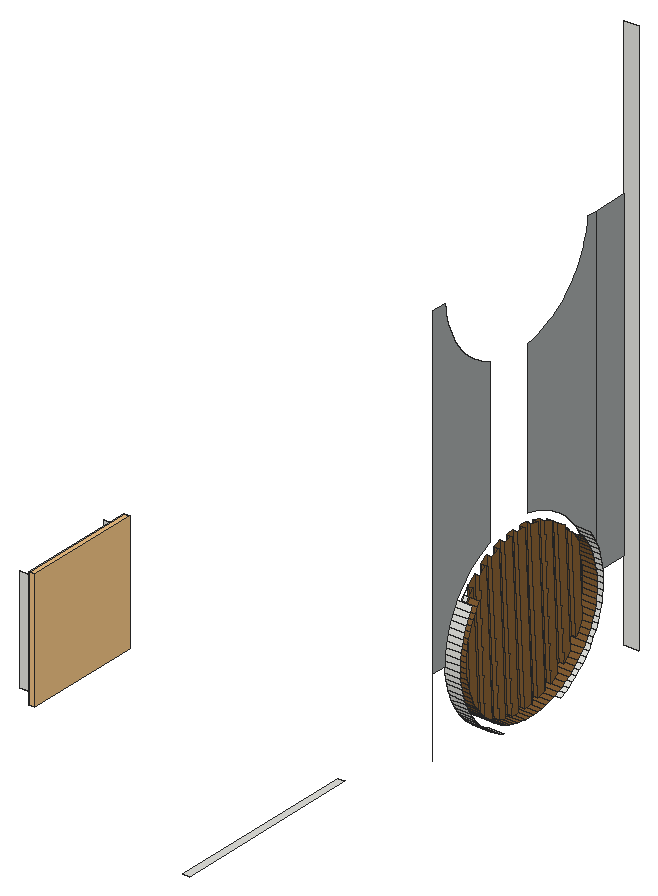
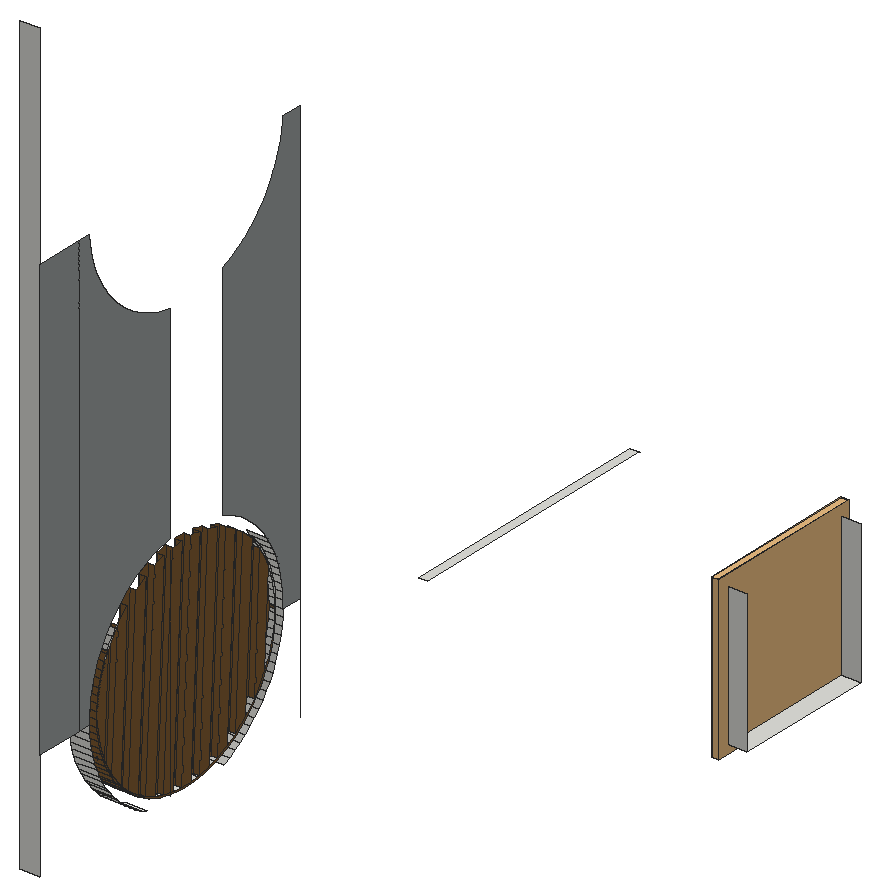
# SketchUp Ruby script. Lengths in inches.
U = 1.inch
M = Sketchup.active_model
def pt(a) = Geom::Point3d.new(a.map { |v| v * U })
def face(e, loops, mat)
  f = e.add_face(loops[0].map { |a| pt(a) })
  loops[1..].each { |l| e.add_face(l.map { |a| pt(a) }).erase! }
  f.material = f.back_material = mat if mat
  f
end
# faces: each face lists its corners as indices into pts; further lists are holes
def faces(e, pts, list, mat = nil) = list.each { |f| face(e, (f[0].is_a?(Array) ? f : [f]).map { |l| l.map { |i| pts[i] } }, mat) }
# xy, xz, yz: faces in a plane at the given z, y or x. An outline is a flat list of corners, or four numbers for a rectangle; further outlines are holes
def ring(l) = l.size == 4 ? [[l[0], l[1]], [l[2], l[1]], [l[2], l[3]], [l[0], l[3]]] : l.each_slice(2).to_a
def flat(e, list, mat, &to3) = list.each { |f| face(e, (f[0].is_a?(Array) ? f : [f]).map { |l| ring(l).map { |u, v| to3.(u, v) } }, mat) }
def xy(e, z, list, mat = nil) = flat(e, list, mat) { |x, y| [x, y, z] }
def xz(e, y, list, mat = nil) = flat(e, list, mat) { |x, z| [x, y, z] }
def yz(e, x, list, mat = nil) = flat(e, list, mat) { |y, z| [x, y, z] }
def lines(e, pts, list) = list.each { |a, b| e.add_line(pt(pts[a]), pt(pts[b])) }
# prism: a flat outline (further loops are holes) pulled along v
def prism(e, loops, v, mat = nil)
  f = face(e, loops, mat); d = Geom::Vector3d.new(v.map { |x| x * U })
  f.pushpull(f.normal.samedirection?(d) ? d.length : -d.length)
end
def box(e, o, s, mat = nil) = prism(e, [[o, [o[0] + s[0], o[1], o[2]], [o[0] + s[0], o[1] + s[1], o[2]], [o[0], o[1] + s[1], o[2]]]], [0, 0, s[2]], mat)
def at(x, y, z, deg = 0) = Geom::Transformation.translation(pt([x, y, z])) * Geom::Transformation.rotation(ORIGIN, Z_AXIS, deg.degrees)
def axes(o, x, y, z) = Geom::Transformation.new([*x, 0, *y, 0, *z, 0, *pt(o).to_a, 1])
def part(name) = M.definitions.add(name)
# library, detail: a bought-in or finely detailed component or shape, given as its bounding box
def library(name, o, s) = part(name).tap { |d| box(d.entities, o, s) }
def detail(e, o, s) = box(e.add_group.entities, o, s)
def put(e, d, t, mat = nil) = e.add_instance(d, t).tap { |i| i.material = mat if mat }
def group(e, t, mat = nil) = e.add_group.tap { |g| g.transformation = t; g.material = mat if mat }.entities
root = M.entities
M.materials.add("C08_Toffee_Ember").color = [130, 92, 50]
M.materials.add("Denim_03_1K").color = [156, 160, 160]
c1 = library("mesh-165",[-1596.32,-2661.67,-39.91],[1702.88,1739.15,82.5])
c2 = part("Group15")
put(c2.entities,c1,at(294.66,859.51,3.5))
xy(root,168,[[317.82,21,320.5,99]])
xy(root,171,[[206.5,78,212.5,120]])
xz(root,78,[[206.5,171,212.5,213]])
xz(root,120,[[206.5,171,212.5,213]])
xz(root,156.01,[[317.5,186.29,319.5,186.76]])
xz(root,243,[[317.5,153,323.5,378]])
yz(root,212.5,[[[75,168,123,216],[78,171,120,213]]])
yz(root,317.5,[[221.99,185.81,222,186.07,221.97,187.24],[156.01,186.29,156.01,186.76,156.12,188.83,156.36,190.89,156.74,192.93,157.23,194.9375,157.86,196.92,158.6,198.85,158.62,198.88,158.6,199.26,158.46,198.9375,157.73,197,157.13,195.01,156.66,192.99,156.31,190.95,156.09,188.89,156,186.82],[221.97,187.33,221.96,188.14,221.78,190.21,221.48,192.26,221.05,194.29,220.5,196.29,219.82,198.25,219.02,200.16,218.1,202.01,217.92,202.32,217.95,201.82,218.28,201.23,219.17,199.36,219.95,197.44,220.61,195.47,221.14,193.47,221.55,191.4375,221.83,189.38],[158.62,198.88,159.47,200.73,160.45,202.56,161.55,204.32,161.64,204.4375,161.62,204.84,161.34,204.44,160.26,202.67,159.3,200.83,158.6,199.26],[217.95,201.82,217.92,202.32,217.0625,203.8125,215.91,205.54,214.66,207.19,214.35,207.56,214.37,207.08,214.9,206.45,216.14,204.78,217.26,203.04],
  [161.64,204.4375,162.76,206.01,164.0625,207.61,164.74,208.35,164.72,208.77,163.8125,207.76,162.52,206.14,161.62,204.84]])
yz(root,317.5,[[188.24,153.01,190.31,153.03,192.38,153.17,194.4375,153.45,194.92,153.55,194.92,153.98,194.82,153.96,193.99,153.84,192.77,153.66,190.7,153.49,188.63,153.45,187.4,153.5,186.56,153.53,184.49,153.75,184.07,153.82,182.45,154.1,180.73,154.5,180.43,154.58,178.45,155.18,177.375,155.58,176.51,155.9,174.61,156.75,173.99,157.07,172.78,157.71,171,158.78,170.59,159.07,169.3,159.97,167.68,161.26,167.14,161.74,166.14,162.64,164.69,164.125,163.65,165.33,163.34,165.7,162.09,167.35,160.9375,169.08,160.08,170.57,159.9,170.875,158.98,172.73,158.18,174.64,157.5,176.6,156.95,178.6,156.52,180.625,156.22,182.68,156.04,184.74,156.01,186.29,156.03,184.69,156.17,182.62,156.45,180.5625,156.86,178.53,157.39,176.53,158.05,174.56,158.83,172.64,159.72,170.77,160.74,168.96,161.86,167.22,163.1,165.55,164.43,163.97,165.86,162.47,167.39,161.0625,168.99,159.76,170.68,158.55,172.44,157.45,174.27,156.47,176.15,155.6,178.08,154.86,180.0625,154.23,182.07,153.74,184.11,153.36,186.17,153.12],[188.63,153.45,190.7,153.49,187.32,218.95,185.62,218.83,184.04,218.61,187.4,153.5],[194.92,153.55,196.47,153.86,198.47,154.39,200.44,155.05,202.36,155.83,204.23,156.72,206.04,157.74,207.78,158.86,209.45,160.1,211.03,161.43,212.53,162.86,213.9375,164.39,215.24,165.99,216.45,167.68,217.55,169.44,218.53,171.27,219.4,173.15,220.14,175.08,220.77,177.0625,221.26,179.07,221.64,181.11,221.88,183.17,221.99,185.24,221.99,185.81,221.91,184,221.69,181.9375,221.34,179.9,220.87,177.88,220.27,175.89,219.54,173.95,219.4,173.63,218.7,172.06,217.74,170.22,216.66,168.45,216.38,168.05,215.48,166.75,214.1875,165.125,213.28,164.12,212.8,163.58,211.32,162.13,210.13,161.11,209.75,160.78,208.09,159.53,206.95,158.77,206.37,158.38,204.57,157.35,203.74,156.9375,202.71,156.43,200.8,155.625,200.51,155.52,198.84,154.95,197.26,154.5,196.85,154.39,194.92,153.98],[184.07,153.82,180.77,217.94,179.53,217.61,177.56,216.95,177.51,216.93,180.73,154.5,182.45,154.1],[193.99,153.84,194.82,153.96,194.92,153.98,194.92,199.87,193.95,218.625,193.89,218.64,191.83,218.88,190.63,218.94],
  [194.92,153.98,196.85,154.39,197.26,154.5,194.92,199.87],[200.51,155.52,200.8,155.625,202.71,156.43,203.74,156.9375,200.65,216.86,199.92,217.14,197.9375,217.77,197.29,217.93],[177.375,155.58,174.28,215.52,173.77,215.28,171.96,214.26,171.07,213.6875,173.99,157.07,174.61,156.75,176.51,155.9],[206.95,158.77,208.09,159.53,209.75,160.78,210.13,161.11,207.4375,213.36,207.32,213.45,205.56,214.55,204.03,215.37],[170.59,159.07,167.89,211.34,166.97,210.57,165.47,209.14,164.74,208.35,167.14,161.74,167.68,161.26,169.3,159.97],
  [213.28,164.12,214.1875,165.125,215.48,166.75,216.38,168.05,214.37,207.08,213.57,208.03,212.14,209.53,210.88,210.69],[163.65,165.33,161.64,204.4375,161.55,204.32,160.45,202.56,159.47,200.73,158.62,198.88,160.08,170.57,160.9375,169.08,162.09,167.35,163.34,165.7],[219.4,173.63,219.54,173.95,220.27,175.89,220.87,177.88,221.34,179.9,221.69,181.9375,221.91,184,221.99,185.81,221.97,187.24,221.97,187.33,221.83,189.38,221.55,191.4375,221.14,193.47,220.61,195.47,219.95,197.44,219.17,199.36,218.28,201.23,217.95,201.82]],"C08_Toffee_Ember")
yz(root,317.5,[[147,184.57,153.03,184.57,153.01,186.83,153.13,189.09,153.4,191.33,153.8,193.56,154.35,195.75,155.03,197.91,155.84,200.02,156.79,202.07,157.86,204.0625,159.06,205.98,160.37,207.82,161.8,209.58,163.33,211.24,164.97,212.8,166.7,214.26,168.51,215.6,170.41,216.83,172.39,217.9375,174.42,218.92,175.37,219.3,175.37,284.68,174.17,285.22,173.31,285.6,171.3,286.65,170.77,286.97,169.37,287.82,167.51,289.12,167.35,289.24,165.74,290.52,164.0625,292.04,163.9,292.21,162.48,293.65,161,295.37,160.39,296.18,159.64,297.17,158.39,299.05,157.26,301.01,156.78,301.98,156.26,303.04,155.38,305.125,154.64,307.26,154.03,309.44,153.5625,311.65,153.24,313.89,153.12,315.33,147,315.33],[224.99,185.17,228.75,185.17,228.75,315.33,224.9,315.33,224.66,313.09,224.28,310.86,223.77,308.65,223.11,306.49,222.7,305.375,222.32,304.37,221.4,302.31,220.35,300.3,219.71,299.24,219.18,298.37,217.88,296.51,216.625,294.93,216.48,294.74,214.96,293.0625,213.49,291.625,213.35,291.48,211.63,290,210.32,289.01,209.83,288.64,207.95,287.39,207.125,286.92,205.99,286.26,203.96,285.26,201.875,284.38,199.74,283.64,197.56,283.03,195.35,282.5625,194.92,282.5,194.92,221.5,196.56,221.2,198.75,220.65,200.91,219.97,203.02,219.16,205.07,218.21,207.0625,217.14,208.98,215.94,210.82,214.63,212.58,213.2,214.24,211.67,215.8,210.03,217.26,208.3,218.6,206.49,219.83,204.59,220.9375,202.61,221.92,200.58,222.77,198.48,223.48,196.33,224.07,194.15,224.51,191.93,224.81,189.69,224.97,187.43],[228.75,185.17,243,315.33]],"Denim_03_1K")
yz(root,319.5,[[190.7,153.49,192.77,153.66,193.99,153.84,190.63,218.94,189.76,218.99,187.69,218.97,187.32,218.95],[187.4,153.5,184.04,218.61,183.5625,218.55,181.53,218.14,180.77,217.94,184.07,153.82,184.49,153.75,186.56,153.53],[180.73,154.5,177.51,216.93,175.64,216.17,174.28,215.52,177.375,155.58,178.45,155.18,180.43,154.58],[197.26,154.5,198.84,154.95,200.51,155.52,197.29,217.93,195.93,218.26,193.95,218.625],[203.74,156.9375,204.57,157.35,206.37,158.38,206.95,158.77,204.03,215.37,203.73,215.53,201.85,216.4,200.65,216.86],
  [173.99,157.07,171.07,213.6875,170.22,213.14,168.55,211.9,167.89,211.34,170.59,159.07,171,158.78,172.78,157.71],[210.13,161.11,211.32,162.13,212.8,163.58,213.28,164.12,210.88,210.69,210.61,210.9375,209.01,212.24,207.4375,213.36],[167.14,161.74,164.74,208.35,164.0625,207.61,162.76,206.01,161.64,204.4375,163.65,165.33,164.69,164.125,166.14,162.64],[216.38,168.05,216.66,168.45,217.74,170.22,218.7,172.06,219.4,173.63,217.95,201.82,217.26,203.04,216.14,204.78,214.9,206.45,214.37,207.08],[160.08,170.57,158.62,198.88,158.6,198.85,157.86,196.92,157.23,194.9375,156.74,192.93,156.36,190.89,156.12,188.83,156.01,186.76,156.01,186.29,156.04,184.74,156.22,182.68,156.52,180.625,156.95,178.6,157.5,176.6,158.18,174.64,158.98,172.73,159.9,170.875]],"C08_Toffee_Ember")
p = [[317.5,172.93,153.79],[317.5,174.98,152.84],[323.5,174.98,152.84],[323.5,172.93,153.79],[317.5,188.24,153.01],[317.5,186.17,153.12],
  [323.5,186.17,153.12],[323.5,188.24,153.01],[317.5,190.31,153.03],[323.5,190.31,153.03],[317.5,192.38,153.17],[323.5,192.38,153.17],
  [317.5,184.11,153.36],[323.5,184.11,153.36],[317.5,203.58,153.08],[317.5,205.61,154.0625],[323.5,205.61,154.0625],[323.5,203.58,153.08],
  [317.5,194.4375,153.45],[323.5,194.4375,153.45],[317.5,182.07,153.74],[323.5,182.07,153.74],[317.5,187.4,153.5],[317.5,184.04,218.61],
  [319.5,184.04,218.61],[319.5,187.4,153.5],[317.5,184.49,153.75],[317.5,186.56,153.53],[319.5,186.56,153.53],[319.5,184.49,153.75],
  [317.5,187.32,218.95],[317.5,190.7,153.49],[319.5,190.7,153.49],[319.5,187.32,218.95],[317.5,192.77,153.66],[319.5,192.77,153.66],
  [317.5,196.47,153.86],[317.5,194.92,153.55],[323.5,196.47,153.86],[317.5,180.0625,154.23],[323.5,180.0625,154.23],[317.5,193.99,153.84],
  [319.5,193.99,153.84],[317.5,170.9375,154.86],[323.5,170.9375,154.86],[317.5,180.77,217.94],[317.5,184.07,153.82],[319.5,184.07,153.82],
  [319.5,180.77,217.94],[317.5,190.63,218.94],[319.5,190.63,218.94],[317.5,198.47,154.39],[323.5,198.47,154.39],[317.5,207.59,155.17],
  [323.5,207.59,155.17],[317.5,178.08,154.86],[323.5,178.08,154.86],[317.5,200.44,155.05],[323.5,200.44,155.05],[317.5,180.73,154.5],
  [317.5,177.51,216.93],[319.5,177.51,216.93],[319.5,180.73,154.5],[317.5,180.43,154.58],[319.5,180.43,154.58],[317.5,193.95,218.625],
  [317.5,194.92,199.87],[317.5,197.26,154.5],[319.5,197.26,154.5],[319.5,193.95,218.625],[317.5,198.84,154.95],[319.5,198.84,154.95],
  [317.5,178.45,155.18],[319.5,178.45,155.18],[317.5,169.02,156.06],[323.5,169.02,156.06],[317.5,176.15,155.6],[323.5,176.15,155.6],
  [317.5,200.51,155.52],[319.5,200.51,155.52],[317.5,202.36,155.83],[323.5,202.36,155.83],[317.5,177.375,155.58],[319.5,177.375,155.58],
  [317.5,209.49,156.4],[323.5,209.49,156.4],[317.5,197.29,217.93],[319.5,197.29,217.93],[317.5,174.28,215.52],[319.5,174.28,215.52],
  [317.5,174.27,156.47],[323.5,174.27,156.47],[317.5,204.23,156.72],[323.5,204.23,156.72],[317.5,167.18,157.37],[323.5,167.18,157.37],
  [317.5,211.3,157.74],[323.5,211.3,157.74],[317.5,172.44,157.45],[323.5,172.44,157.45],[317.5,206.04,157.74],[323.5,206.04,157.74],
  [317.5,200.65,216.86],[317.5,203.74,156.9375],[319.5,203.74,156.9375],[319.5,200.65,216.86],[317.5,204.57,157.35],[319.5,204.57,157.35],
  [317.5,173.99,157.07],[317.5,171.07,213.6875],[319.5,171.07,213.6875],[319.5,173.99,157.07],[317.5,172.78,157.71],[319.5,172.78,157.71],
  [317.5,206.37,158.38],[319.5,206.37,158.38],[317.5,165.42,158.8],[323.5,165.42,158.8],[317.5,170.68,158.55],[323.5,170.68,158.55],
  [317.5,171,158.78],[319.5,171,158.78],[317.5,207.78,158.86],[323.5,207.78,158.86],[317.5,213.03,159.2],[323.5,213.03,159.2],
  [317.5,206.95,158.77],[319.5,206.95,158.77],[317.5,168.99,159.76],[323.5,168.99,159.76],[317.5,163.76,160.33],[323.5,163.76,160.33],
  [317.5,170.59,159.07],[319.5,170.59,159.07],[317.5,204.03,215.37],[319.5,204.03,215.37],[317.5,209.45,160.1],[323.5,209.45,160.1],
  [317.5,167.89,211.34],[319.5,167.89,211.34],[317.5,214.67,160.76],[323.5,214.67,160.76],[317.5,167.39,161.0625],[323.5,167.39,161.0625],
  [317.5,211.03,161.43],[323.5,211.03,161.43],[317.5,162.2,161.97],[323.5,162.2,161.97],[317.5,216.2,162.42],[323.5,216.2,162.42],
  [317.5,165.86,162.47],[323.5,165.86,162.47],[317.5,207.4375,213.36],[317.5,210.13,161.11],[319.5,210.13,161.11],[319.5,207.4375,213.36],
  [317.5,211.32,162.13],[319.5,211.32,162.13],[317.5,212.53,162.86],[323.5,212.53,162.86],[317.5,167.14,161.74],[317.5,164.74,208.35],
  [319.5,164.74,208.35],[319.5,167.14,161.74],[317.5,166.14,162.64],[319.5,166.14,162.64],[317.5,160.74,163.7],[323.5,160.74,163.7],
  [317.5,212.8,163.58],[319.5,212.8,163.58],[317.5,217.63,164.18],[323.5,217.63,164.18],[317.5,164.43,163.97],[323.5,164.43,163.97],
  [317.5,164.69,164.125],[319.5,164.69,164.125],[317.5,213.9375,164.39],[323.5,213.9375,164.39],[317.5,213.28,164.12],[319.5,213.28,164.12],
  [317.5,159.4,165.51],[323.5,159.4,165.51],[317.5,163.1,165.55],[323.5,163.1,165.55],[317.5,163.65,165.33],[319.5,163.65,165.33],
  [317.5,210.88,210.69],[319.5,210.88,210.69],[317.5,218.94,166.02],[323.5,218.94,166.02],[317.5,215.24,165.99],[323.5,215.24,165.99],
  [317.5,161.64,204.4375],[319.5,161.64,204.4375],[317.5,158.17,167.41],[323.5,158.17,167.41],[317.5,161.86,167.22],[323.5,161.86,167.22],
  [317.5,216.45,167.68],[323.5,216.45,167.68],[317.5,220.14,167.9375],[323.5,220.14,167.9375],[317.5,160.74,168.96],[323.5,160.74,168.96],
  [317.5,157.0625,169.39],[323.5,157.0625,169.39],[317.5,217.55,169.44],[323.5,217.55,169.44],[317.5,221.21,169.93],[323.5,221.21,169.93],
  [317.5,214.37,207.08],[317.5,216.38,168.05],[319.5,216.38,168.05],[319.5,214.37,207.08],[317.5,216.66,168.45],[319.5,216.66,168.45],
  [317.5,217.74,170.22],[319.5,217.74,170.22],[317.5,159.72,170.77],[323.5,159.72,170.77],[317.5,156.08,171.42],[323.5,156.08,171.42],
  [317.5,218.53,171.27],[323.5,218.53,171.27],[317.5,222.16,171.98],[323.5,222.16,171.98],[317.5,218.7,172.06],[319.5,218.7,172.06],
  [317.5,160.08,170.57],[317.5,158.62,198.88],[319.5,158.62,198.88],[319.5,160.08,170.57],[317.5,159.9,170.875],[319.5,159.9,170.875],
  [317.5,158.83,172.64],[323.5,158.83,172.64],[317.5,158.98,172.73],[319.5,158.98,172.73],[317.5,219.4,173.15],[323.5,219.4,173.15],
  [317.5,155.23,173.52],[323.5,155.23,173.52],[317.5,222.97,174.09],[323.5,222.97,174.09],[317.5,219.4,173.63],[319.5,219.4,173.63],
  [317.5,158.05,174.56],[323.5,158.05,174.56],[317.5,158.18,174.64],[319.5,158.18,174.64],[317.5,220.14,175.08],[323.5,220.14,175.08],
  [317.5,154.52,175.67],[323.5,154.52,175.67],[317.5,217.95,201.82],[319.5,217.95,201.82],[317.5,223.65,176.25],[323.5,223.65,176.25],
  [317.5,157.39,176.53],[323.5,157.39,176.53],[317.5,157.5,176.6],[319.5,157.5,176.6],[317.5,220.77,177.0625],[323.5,220.77,177.0625],
  [317.5,153.93,177.85],[323.5,153.93,177.85],[317.5,224.2,178.44],[323.5,224.2,178.44],[317.5,156.86,178.53],[323.5,156.86,178.53],
  [317.5,156.95,178.6],[319.5,156.95,178.6],[317.5,221.26,179.07],[323.5,221.26,179.07],[317.5,153.49,180.07],[323.5,153.49,180.07],
  [317.5,224.6,180.67],[323.5,224.6,180.67],[317.5,156.45,180.5625],[323.5,156.45,180.5625],[317.5,156.52,180.625],[319.5,156.52,180.625],
  [317.5,221.64,181.11],[323.5,221.64,181.11],[317.5,153.19,182.31],[323.5,153.19,182.31],[317.5,156.17,182.62],[323.5,156.17,182.62],
  [317.5,156.22,182.68],[319.5,156.22,182.68],[317.5,224.87,182.91],[323.5,224.87,182.91],[317.5,221.88,183.17],[323.5,221.88,183.17],
  [317.5,153.03,184.57],[323.5,153.03,184.57],[317.5,156.03,184.69],[323.5,156.03,184.69],[317.5,156.04,184.74],[319.5,156.04,184.74],
  [317.5,224.99,185.17],[323.5,224.99,185.17],[317.5,221.99,185.24],[323.5,221.99,185.24],[317.5,153.01,186.83],[323.5,153.01,186.83],
  [317.5,156.01,186.29],[319.5,156.01,186.29],[319.5,156.01,186.76],[323.5,156.01,186.76],[317.5,221.97,187.31],[317.5,221.97,187.24],
  [317.5,221.99,185.81],[323.5,221.97,187.31],[317.5,224.97,187.43],[323.5,224.97,187.43],[317.5,153.13,189.09],[323.5,153.13,189.09],
  [317.5,156.01,186.76],[317.5,156.12,188.83],[319.5,156.12,188.83],[323.5,156.12,188.83],[317.5,221.83,189.38],[317.5,221.97,187.33],
  [323.5,221.83,189.38],[317.5,224.81,189.69],[323.5,224.81,189.69],[317.5,156.36,190.89],[319.5,156.36,190.89],[323.5,156.36,190.89],
  [317.5,153.4,191.33],[323.5,153.4,191.33],[317.5,221.55,191.4375],[323.5,221.55,191.4375],[317.5,224.51,191.93],[323.5,224.51,191.93],
  [317.5,156.74,192.93],[319.5,156.74,192.93],[323.5,156.74,192.93],[317.5,153.8,193.56],[323.5,153.8,193.56],[317.5,221.14,193.47],
  [323.5,221.14,193.47],[317.5,224.07,194.15],[323.5,224.07,194.15],[317.5,157.23,194.9375],[319.5,157.23,194.9375],[323.5,157.23,194.9375],
  [317.5,220.61,195.47],[323.5,220.61,195.47],[317.5,154.35,195.75],[323.5,154.35,195.75],[317.5,223.48,196.33],[323.5,223.48,196.33],
  [317.5,157.86,196.92],[319.5,157.86,196.92],[323.5,157.86,196.92],[317.5,219.95,197.44],[323.5,219.95,197.44],[317.5,155.03,197.91],
  [323.5,155.03,197.91],[317.5,222.77,198.48],[323.5,222.77,198.48],[317.5,158.6,198.85],[319.5,158.6,198.85],[323.5,158.6,198.85],
  [317.5,219.17,199.36],[323.5,219.17,199.36],[317.5,155.84,200.02],[323.5,155.84,200.02],[317.5,221.92,200.58],[323.5,221.92,200.58],
  [317.5,159.47,200.73],[323.5,159.47,200.73],[317.5,218.28,201.23],[323.5,218.28,201.23],[317.5,156.79,202.07],[323.5,156.79,202.07],
  [317.5,220.9375,202.61],[323.5,220.9375,202.61],[317.5,160.45,202.56],[323.5,160.45,202.56],[323.5,217.26,203.04],[319.5,217.26,203.04],
  [317.5,217.26,203.04],[317.5,157.86,204.0625],[323.5,157.86,204.0625],[317.5,161.55,204.32],[323.5,161.55,204.32],[317.5,219.83,204.59],
  [323.5,219.83,204.59],[317.5,216.14,204.78],[319.5,216.14,204.78],[323.5,216.14,204.78],[317.5,159.06,205.98],[323.5,159.06,205.98],
  [319.5,162.76,206.01],[323.5,162.76,206.01],[317.5,162.76,206.01],[317.5,218.6,206.49],[323.5,218.6,206.49],[317.5,214.9,206.45],
  [319.5,214.9,206.45],[323.5,214.9,206.45],[317.5,21,168],[317.82,21,168],[317.5,194.92,153],[317.5,194.92,218.45],
  [317.5,146.83,153],[317.5,146.83,252]]
faces(root,p,[[0,1,2,3],[14,15,16,17],[26,27,28,29],[27,22,25,28],[31,34,35,32],[34,41,42,35],[43,0,3,44],[46,26,29,47],
  [15,53,54,16],[63,59,62,64],[67,70,71,68],[72,63,64,73],[74,43,44,75],[70,78,79,71],[82,72,73,83],[53,84,85,54],
  [94,74,75,95],[84,96,97,85],[103,106,107,104],[112,108,111,113],[106,114,115,107],[116,94,95,117],[120,112,113,121],[96,124,125,97],
  [114,126,127,115],[130,116,117,131],[132,120,121,133],[124,140,141,125],[146,130,131,147],[140,148,149,141],[153,156,157,154],[164,160,163,165],
  [166,146,147,167],[156,168,169,157],[148,170,171,149],[174,164,165,175],[168,178,179,169],[180,166,167,181],[184,174,175,185],[170,188,189,171],
  [194,180,181,195],[188,200,201,189],[204,194,195,205],[200,208,209,201],[211,214,215,212],[214,216,217,215],[220,204,205,221],[208,224,225,209],
  [216,226,227,217],[232,228,231,233],[236,232,233,237],[240,220,221,241],[224,242,243,225],[226,244,245,227],[248,236,237,249],[252,240,241,253],
  [242,256,257,243],[260,248,249,261],[264,252,253,265],[256,266,267,257],[270,260,261,271],[274,264,265,275],[266,276,277,267],[280,270,271,281],
  [284,274,275,285],[288,280,281,289],[276,290,291,277],[294,284,285,295],[298,288,289,299],[290,300,301,291],[304,294,295,305],[306,298,299,307],
  [300,314,315,301],[316,304,305,317],[318,319,320,308],[314,325,326,315],[319,327,328,320],[330,316,317,331],[325,334,335,326],[327,336,337,328],
  [339,330,331,340],[334,343,344,335],[336,345,346,337],[350,339,340,351],[343,352,353,344],[345,354,355,346],[359,350,351,360],[352,361,362,353],
  [354,363,364,355],[368,359,360,369],[361,370,371,362],[363,229,230,364],[376,368,369,377],[370,378,379,371],[384,254,255,383],[385,376,377,386],
  [378,389,390,379],[391,384,383,392],[394,385,386,395],[192,398,396,193],[389,399,400,390],[401,391,392,402]])
faces(root,p,[[4,5,6,7],[8,4,7,9],[10,8,9,11],[5,12,13,6],[18,10,11,19],[12,20,21,13],[22,23,24,25],[30,31,32,33],
  [36,37,18,19,38],[20,39,40,21],[45,46,47,48],[41,49,50,42],[51,36,38,52],[39,55,56,40],[57,51,52,58],[59,60,61,62],
  [65,66,67,68,69],[55,76,77,56],[80,57,58,81],[78,86,87,79],[88,82,83,89],[76,90,91,77],[92,80,81,93],[90,98,99,91],
  [100,92,93,101],[102,103,104,105],[108,109,110,111],[98,118,119,99],[122,100,101,123],[118,128,129,119],[126,134,135,127],[136,122,123,137],
  [138,132,133,139],[128,142,143,129],[144,136,137,145],[142,150,151,143],[152,153,154,155],[158,144,145,159],[160,161,162,163],[150,172,173,151],
  [176,158,159,177],[172,182,183,173],[178,186,187,179],[190,176,177,191],[192,184,185,193],[182,196,197,183],[198,190,191,199],[196,202,203,197],
  [206,198,199,207],[210,211,212,213],[202,218,219,203],[222,206,207,223],[228,229,230,231],[218,234,235,219],[238,222,223,239],[234,246,247,235],
  [250,238,239,251],[244,254,255,245],[246,258,259,247],[262,250,251,263],[258,268,269,259],[272,262,263,273],[268,278,279,269],[282,272,273,283],
  [278,286,287,279],[292,282,283,293],[286,296,297,287],[302,292,293,303],[296,306,307,308,309,297],[310,311,312,302,303,313],[309,308,320,321],[322,323,310,313,324],
  [321,320,328,329],[332,322,324,333],[329,328,337,338],[341,332,333,342],[338,337,346,347],[348,341,342,349],[347,346,355,356],[357,348,349,358],
  [356,355,364,365],[366,357,358,367],[365,364,230,229,372,373],[374,366,367,375],[372,380,381,373],[382,383,255,254,374,375],[380,387,388,381],[393,392,383,382],
  [387,192,193,396,397,388],[403,402,392,393]],"C08_Toffee_Ember")
lines(root,p,[[404,405],[406,37],[66,407],[408,409]])
put(root,c2,axes([213.625,86.43,217.74],[0,-0.02811,0],[0,0,0.02756],[-0.02756,0,0]))
